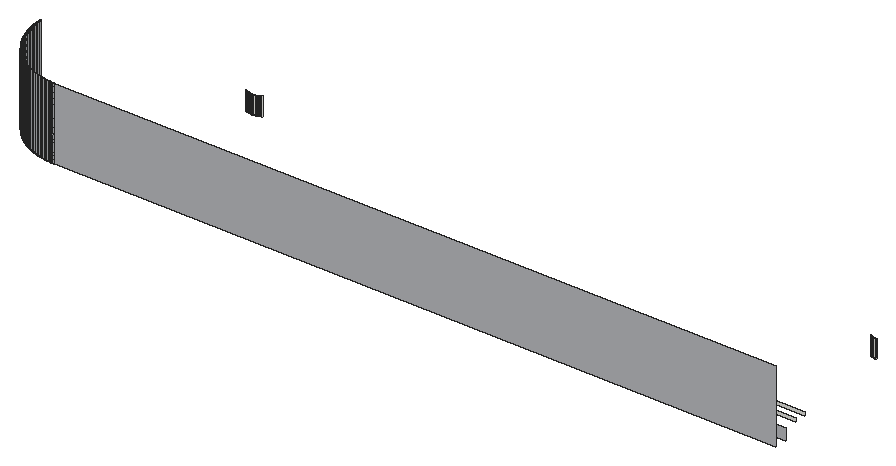
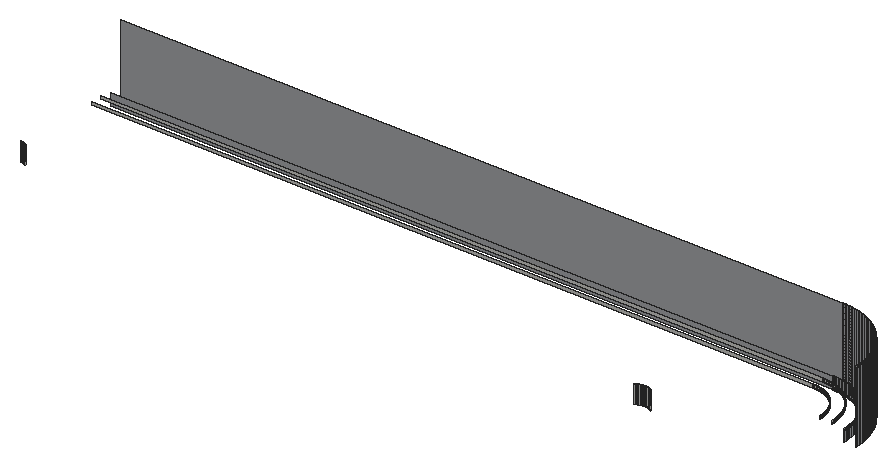
# SketchUp Ruby script. Lengths in inches.
U = 1.inch
M = Sketchup.active_model
def pt(a) = Geom::Point3d.new(a.map { |v| v * U })
def face(e, loops, mat)
  f = e.add_face(loops[0].map { |a| pt(a) })
  loops[1..].each { |l| e.add_face(l.map { |a| pt(a) }).erase! }
  f.material = f.back_material = mat if mat
  f
end
# faces: each face lists its corners as indices into pts; further lists are holes
def faces(e, pts, list, mat = nil) = list.each { |f| face(e, (f[0].is_a?(Array) ? f : [f]).map { |l| l.map { |i| pts[i] } }, mat) }
# xy, xz, yz: faces in a plane at the given z, y or x. An outline is a flat list of corners, or four numbers for a rectangle; further outlines are holes
def ring(l) = l.size == 4 ? [[l[0], l[1]], [l[2], l[1]], [l[2], l[3]], [l[0], l[3]]] : l.each_slice(2).to_a
def flat(e, list, mat, &to3) = list.each { |f| face(e, (f[0].is_a?(Array) ? f : [f]).map { |l| ring(l).map { |u, v| to3.(u, v) } }, mat) }
def xy(e, z, list, mat = nil) = flat(e, list, mat) { |x, y| [x, y, z] }
def xz(e, y, list, mat = nil) = flat(e, list, mat) { |x, z| [x, y, z] }
def yz(e, x, list, mat = nil) = flat(e, list, mat) { |y, z| [x, y, z] }
def lines(e, pts, list) = list.each { |a, b| e.add_line(pt(pts[a]), pt(pts[b])) }
# prism: a flat outline (further loops are holes) pulled along v
def prism(e, loops, v, mat = nil)
  f = face(e, loops, mat); d = Geom::Vector3d.new(v.map { |x| x * U })
  f.pushpull(f.normal.samedirection?(d) ? d.length : -d.length)
end
def box(e, o, s, mat = nil) = prism(e, [[o, [o[0] + s[0], o[1], o[2]], [o[0] + s[0], o[1] + s[1], o[2]], [o[0], o[1] + s[1], o[2]]]], [0, 0, s[2]], mat)
def at(x, y, z, deg = 0) = Geom::Transformation.translation(pt([x, y, z])) * Geom::Transformation.rotation(ORIGIN, Z_AXIS, deg.degrees)
def axes(o, x, y, z) = Geom::Transformation.new([*x, 0, *y, 0, *z, 0, *pt(o).to_a, 1])
def part(name) = M.definitions.add(name)
# library, detail: a bought-in or finely detailed component or shape, given as its bounding box
def library(name, o, s) = part(name).tap { |d| box(d.entities, o, s) }
def detail(e, o, s) = box(e.add_group.entities, o, s)
def put(e, d, t, mat = nil) = e.add_instance(d, t).tap { |i| i.material = mat if mat }
def group(e, t, mat = nil) = e.add_group.tap { |g| g.transformation = t; g.material = mat if mat }.entities
root = M.entities
M.materials.add("1427 AP 686 ARMOUR-N").color = [184, 186, 189]
xz(root,129.92,[[21,240,141,252]],"1427 AP 686 ARMOUR-N")
xz(root,129.93,[[20.53,240,20.6875,252],[20.6875,240,20.84,252]],"1427 AP 686 ARMOUR-N")
xz(root,131.92,[[21,240,21.01,242],[21.01,240,140.99,242]],"1427 AP 686 ARMOUR-N")
xz(root,131.93,[[20.61,240,20.74,242],[20.74,240,20.87,242]],"1427 AP 686 ARMOUR-N")
xz(root,133.92,[[21.01,242,140.99,242.5]])
xz(root,133.93,[[20.6875,242,20.79,242.5],[20.79,242,20.9,242.5]])
xz(root,133.94,[[20.48,242,20.58,242.5]])
xz(root,135.92,[[21.02,242,140.98,242.5]])
xz(root,135.93,[[20.6875,242,20.76,242.5],[20.76,242,20.84,242.5],[20.84,242,20.92,242.5]])
xz(root,153.43,[[34.84,242,34.92,245],[35.08,242,35.16,245]])
xz(root,153.44,[[34.6875,242,34.76,245],[35.24,242,35.3125,245],[138.6875,242,138.76,245]])
yz(root,9,[[141.61,240,141.77,252],[141.77,240,141.92,252]],"1427 AP 686 ARMOUR-N")
yz(root,11,[[141.66,240,141.79,242],[141.79,240,141.93,242]],"1427 AP 686 ARMOUR-N")
yz(root,11.01,[[141.4,240,141.53,242]],"1427 AP 686 ARMOUR-N")
yz(root,13,[[141.71,242,141.82,242.5],[141.82,242,141.9375,242.5]])
yz(root,13.01,[[141.51,242,141.61,242.5]])
yz(root,13.02,[[141.3,242,141.4,242.5]])
yz(root,15,[[141.6875,242,141.77,242.5],[141.77,242,141.85,242.5],[141.85,242,141.94,242.5]])
yz(root,15.01,[[141.53,242,141.61,242.5]])
yz(root,15.03,[[141.3,242,141.375,242.5]])
p = [[20.37,129.94,252],[20.22,129.95,252],[20.22,129.95,240],[20.37,129.94,240],[20.53,129.93,252],[20.53,129.93,240],
  [21,129.92,252],[20.84,129.93,252],[20.84,129.93,240],[20.99,129.92,240],[21,129.92,240],[19.28,130.05,252],
  [19.12,130.07,252],[19.12,130.07,240],[19.28,130.05,240],[19.43,130.03,252],[19.43,130.03,240],[19.59,130.01,252],
  [19.59,130.01,240],[19.75,129.99,252],[19.75,129.99,240],[19.9,129.97,252],[19.9,129.97,240],[20.06,129.96,252],
  [20.06,129.96,240],[18.8125,130.125,252],[18.66,130.15,252],[18.66,130.15,240],[18.8125,130.125,240],[18.97,130.1,252],
  [18.97,130.1,240],[18.35,130.22,252],[18.2,130.26,252],[18.2,130.26,240],[18.35,130.22,240],[18.51,130.1875,252],
  [18.51,130.1875,240],[17.89,130.33,252],[17.74,130.375,252],[17.74,130.375,240],[17.89,130.33,240],[18.05,130.29,252],
  [18.05,130.29,240],[17.59,130.42,252],[17.44,130.46,252],[17.44,130.46,240],[17.59,130.42,240],[17.29,130.51,252],
  [17.14,130.5625,252],[17.14,130.5625,240],[17.29,130.51,240],[16.99,130.61,252],[16.85,130.67,252],[16.85,130.67,240],
  [16.99,130.61,240],[16.7,130.72,252],[16.55,130.78,252],[16.55,130.78,240],[16.7,130.72,240],[16.41,130.84,252],
  [16.26,130.9,252],[16.26,130.9,240],[16.41,130.84,240],[16.12,130.96,252],[16.12,130.96,240],[15.98,131.03,252],
  [15.83,131.09,252],[15.83,131.09,240],[15.98,131.03,240],[15.69,131.16,252],[15.69,131.16,240],[15.55,131.23,252],
  [15.41,131.3,252],[15.41,131.3,240],[15.55,131.23,240],[15.27,131.38,252],[15.27,131.38,240],[15.14,131.45,252],
  [15.14,131.45,240],[15,131.53,252],[14.86,131.61,252],[14.86,131.61,240],[15,131.53,240],[14.73,131.69,252],
  [14.73,131.69,240],[14.6,131.78,252],[14.6,131.78,240],[14.46,131.86,252],[14.46,131.86,240],[14.33,131.95,252],
  [14.2,132.03,252],[14.2,132.03,240],[14.33,131.95,240],[20.35,131.95,240],[20.22,131.96,240],[20.22,131.96,242],
  [20.35,131.95,242],[20.48,131.9375,240],[20.48,131.9375,242],[20.61,131.93,240],[20.61,131.93,242],[21,131.92,240],
  [20.87,131.93,240],[20.87,131.93,242],[21,131.92,242],[14.07,132.125,252],[14.07,132.125,240],[19.4375,132.05,240],
  [19.31,132.07,240],[19.31,132.07,242],[19.4375,132.05,242],[19.57,132.03,240],[19.57,132.03,242],[19.69,132.01,240],
  [19.69,132.01,242],[19.82,131.99,240],[19.82,131.99,242],[19.95,131.98,240],[19.95,131.98,242],[20.09,131.97,240],
  [20.09,131.97,242],[13.95,132.22,252],[13.95,132.22,240],[18.92,132.14,240],[18.79,132.17,240],[18.79,132.17,242],
  [18.92,132.14,242],[19.05,132.12,240],[19.05,132.12,242],[19.18,132.09,240],[19.18,132.09,242],[13.82,132.31,252],
  [13.82,132.31,240],[18.54,132.23,240],[18.41,132.27,240],[18.41,132.27,242],[18.54,132.23,242],[18.67,132.2,240],
  [18.67,132.2,242],[13.69,132.4,252],[13.69,132.4,240],[18.16,132.34,240],[18.03,132.375,240],[18.03,132.375,242],
  [18.16,132.34,242],[18.29,132.3,240],[18.29,132.3,242],[13.57,132.5,252],[13.57,132.5,240],[17.91,132.41,240],
  [17.79,132.46,240],[17.79,132.46,242],[17.91,132.41,242],[13.45,132.6,252],[13.45,132.6,240],[17.54,132.54,240],
  [17.42,132.59,240],[17.42,132.59,242],[17.54,132.54,242],[17.66,132.5,240],[17.66,132.5,242],[13.33,132.7,252],
  [13.33,132.7,240],[17.29,132.64,240],[17.17,132.6875,240],[17.17,132.6875,242],[17.29,132.64,242],[13.21,132.8,252],
  [13.21,132.8,240],[17.05,132.74,240],[16.93,132.79,240],[16.93,132.79,242],[17.05,132.74,242],[13.09,132.9,252],
  [13.09,132.9,240],[16.8125,132.84,240],[16.7,132.9,240],[16.7,132.9,242],[16.8125,132.84,242],[12.97,133.01,252],
  [12.97,133.01,240],[16.58,132.96,240],[16.58,132.96,242],[12.85,133.11,252],[12.85,133.11,240],[16.46,133.01,240],
  [16.34,133.07,240],[16.34,133.07,242],[16.46,133.01,242],[12.74,133.22,252],[12.74,133.22,240],[16.23,133.14,240],
  [16.11,133.2,240],[16.11,133.2,242],[16.23,133.14,242],[12.625,133.33,252],[12.625,133.33,240],[16,133.26,240],
  [16,133.26,242],[12.51,133.4375,252],[12.51,133.4375,240],[15.89,133.33,240],[15.78,133.4,240],[15.78,133.4,242],
  [15.89,133.33,242],[12.4,133.55,252],[12.4,133.55,240],[15.66,133.47,240],[15.66,133.47,242],[15.55,133.54,240],
  [15.44,133.61,240],[15.44,133.61,242],[15.55,133.54,242],[12.3,133.66,252],[12.3,133.66,240],[15.34,133.68,240],
  [15.34,133.68,242],[12.1875,133.78,252],[12.1875,133.78,240],[15.23,133.76,240],[15.23,133.76,242],[12.08,133.89,252],
  [12.08,133.89,240],[15.12,133.83,240],[15.02,133.91,240],[15.02,133.91,242],[15.12,133.83,242],[11.98,134.01,252],
  [11.98,134.01,240],[14.91,133.99,240],[14.91,133.99,242],[11.875,134.13,252],[11.875,134.13,240],[14.81,134.07,240],
  [14.81,134.07,242],[11.77,134.25,252],[11.77,134.25,240],[14.71,134.15,240],[14.71,134.15,242],[14.61,134.24,240],
  [14.51,134.32,240],[14.51,134.32,242],[14.61,134.24,242],[11.67,134.37,252],[11.67,134.37,240],[14.41,134.41,240],
  [14.41,134.41,242],[11.58,134.5,252],[11.58,134.5,240],[14.31,134.49,240],[14.31,134.49,242],[11.48,134.62,252],
  [11.48,134.62,240],[14.21,134.58,240],[14.21,134.58,242],[11.39,134.74,252],[11.39,134.74,240],[14.12,134.67,240],
  [14.12,134.67,242],[11.29,134.87,252],[11.29,134.87,240],[14.02,134.76,240],[14.02,134.76,242],[13.93,134.85,240],
  [13.93,134.85,242],[11.2,135,252],[11.2,135,240],[13.84,134.95,240],[13.75,135.04,240],[13.75,135.04,242],
  [13.84,134.95,242],[11.11,135.13,252],[11.11,135.13,240],[13.66,135.14,240],[13.66,135.14,242],[11.02,135.26,252],
  [11.02,135.26,240],[13.57,135.23,240],[13.57,135.23,242],[13.48,135.33,240],[13.48,135.33,242],[10.9375,135.39,252],
  [10.9375,135.39,240],[13.4,135.43,240],[13.4,135.43,242],[10.85,135.52,252],[10.85,135.52,240],[13.3125,135.53,240],
  [13.3125,135.53,242],[10.77,135.65,252],[10.77,135.65,240],[13.23,135.63,240],[13.23,135.63,242],[13.15,135.73,240],
  [13.15,135.73,242],[10.6875,135.79,252],[10.6875,135.79,240],[13.07,135.84,240],[13.07,135.84,242],[10.61,135.92,252],
  [10.61,135.92,240],[12.99,135.94,240],[12.99,135.94,242],[10.53,136.0625,252],[10.53,136.0625,240],[12.91,136.05,240],
  [12.91,136.05,242],[12.83,136.15,240],[12.83,136.15,242],[10.45,136.2,252],[10.45,136.2,240],[10.38,136.34,252],
  [10.38,136.34,240],[12.76,136.26,240],[12.76,136.26,242],[10.31,136.48,252],[10.31,136.48,240],[12.69,136.37,240],
  [12.69,136.37,242],[12.61,136.48,240],[12.61,136.48,242],[10.24,136.62,252],[10.24,136.62,240],[12.54,136.59,240],
  [12.54,136.59,242],[10.17,136.76,252],[10.17,136.76,240],[12.47,136.7,240],[12.47,136.7,242],[12.41,136.8125,240],
  [12.41,136.8125,242],[10.1,136.9,252],[10.1,136.9,240],[12.34,136.92,240],[12.34,136.92,242],[10.04,137.04,252],
  [10.04,137.04,240],[12.28,137.04,240],[12.28,137.04,242],[9.97,137.1875,252],[9.97,137.1875,240],[12.21,137.15,240],
  [12.21,137.15,242],[9.91,137.33,252],[9.91,137.33,240],[12.15,137.27,240],[12.15,137.27,242],[9.85,137.48,252],
  [9.85,137.48,240],[12.09,137.38,240],[12.09,137.38,242],[12.03,137.5,240],[12.03,137.5,242],[9.8,137.625,252],
  [9.8,137.625,240],[11.97,137.62,240],[11.97,137.62,242],[9.74,137.77,252],[9.74,137.77,240],[11.92,137.74,240],
  [11.92,137.74,242],[11.86,137.86,240],[11.86,137.86,242],[9.6875,137.92,252],[9.6875,137.92,240],[9.64,138.07,252],
  [9.64,138.07,240],[11.8125,137.98,240],[11.8125,137.98,242],[11.76,138.1,240],[11.76,138.1,242],[9.59,138.22,252],
  [9.59,138.22,240],[11.71,138.22,240],[11.71,138.22,242],[9.54,138.37,252],[9.54,138.37,240],[11.66,138.34,240],
  [11.66,138.34,242],[11.62,138.46,240],[11.62,138.46,242],[9.49,138.52,252],[9.49,138.52,240],[9.45,138.67,252],
  [9.45,138.67,240],[11.57,138.59,240],[11.57,138.59,242],[11.53,138.71,240],[11.53,138.71,242],[9.41,138.82,252],
  [9.41,138.82,240],[11.49,138.83,240],[11.49,138.83,242],[9.37,138.97,252],[9.37,138.97,240],[11.45,138.96,240],
  [11.45,138.96,242],[9.33,139.125,252],[9.33,139.125,240],[11.41,139.08,240],[11.41,139.08,242],[9.3,139.28,252],
  [9.3,139.28,240],[11.375,139.21,240],[11.375,139.21,242],[11.34,139.34,240],[11.34,139.34,242],[9.26,139.43,252],
  [9.26,139.43,240],[11.31,139.46,240],[11.31,139.46,242],[9.23,139.58,252],[9.23,139.58,240],[11.28,139.59,240],
  [11.28,139.59,242],[9.2,139.74,252],[9.2,139.74,240],[11.25,139.72,240],[11.25,139.72,242],[9.17,139.89,252],
  [9.17,139.89,240],[11.22,139.85,240],[11.22,139.85,242],[11.19,139.97,240],[11.19,139.97,242],[9.15,140.05,252],
  [9.15,140.05,240],[9.125,140.2,252],[9.125,140.2,240],[11.17,140.1,240],[11.17,140.1,242],[11.14,140.23,240],
  [11.14,140.23,242],[9.1,140.36,252],[9.1,140.36,240],[11.125,140.36,240],[11.125,140.36,242],[9.08,140.51,252],
  [9.08,140.51,240],[11.1,140.49,240],[11.1,140.49,242],[9.07,140.67,252],[9.07,140.67,240],[11.09,140.62,240],
  [11.09,140.62,242],[11.07,140.75,240],[11.07,140.75,242],[9.05,140.83,252],[9.05,140.83,240],[11.05,140.88,240],
  [11.05,140.88,242],[9.04,140.98,252],[9.04,140.98,240],[11.04,141.01,240],[11.04,141.01,242],[9.03,141.14,252],
  [9.03,141.14,240],[11.03,141.14,240],[11.03,141.14,242],[9.02,141.3,252],[9.02,141.3,240],[11.02,141.27,240],
  [11.02,141.27,242],[9.01,141.45,252],[9.01,141.45,240],[11.01,141.4,240],[11.01,141.4,242],[9,141.61,252],
  [9,141.61,240],[11.01,141.53,240],[11,141.66,240],[11,141.66,242],[11.01,141.53,242],[20.37,133.95,242],
  [20.27,133.96,242],[20.27,133.96,242.5],[20.37,133.95,242.5],[20.48,133.94,242],[20.48,133.94,242.5],[20.6875,133.93,242],
  [20.58,133.94,242],[20.58,133.94,242.5],[20.6875,133.93,242.5],[21.01,133.92,242],[20.9,133.93,242],[20.9,133.93,242.5],
  [21.01,133.92,242.5],[19.65,134.04,242],[19.54,134.06,242],[19.54,134.06,242.5],[19.65,134.04,242.5],[19.75,134.02,242],
  [19.75,134.02,242.5],[19.85,134.01,242],[19.85,134.01,242.5],[19.96,133.99,242],[19.96,133.99,242.5],[20.06,133.98,242],
  [20.06,133.98,242.5],[20.16,133.97,242],[20.16,133.97,242.5],[19.13,134.15,242],[19.03,134.17,242],[19.03,134.17,242.5],
  [19.13,134.15,242.5],[19.23,134.12,242],[19.23,134.12,242.5],[19.34,134.1,242],[19.34,134.1,242.5],[19.4375,134.08,242],
  [19.4375,134.08,242.5],[18.83,134.22,242],[18.73,134.25,242],[18.73,134.25,242.5],[18.83,134.22,242.5],[18.93,134.2,242],
  [18.93,134.2,242.5],[18.43,134.35,242],[18.33,134.38,242],[18.33,134.38,242.5],[18.43,134.35,242.5],[18.53,134.32,242],
  [18.53,134.32,242.5],[18.63,134.28,242],[18.63,134.28,242.5],[18.23,134.42,242],[18.13,134.46,242],[18.13,134.46,242.5],
  [18.23,134.42,242.5],[17.9375,134.53,242],[17.84,134.57,242],[17.84,134.57,242.5],[17.9375,134.53,242.5],[18.04,134.49,242],
  [18.04,134.49,242.5],[17.75,134.62,242],[17.65,134.66,242],[17.65,134.66,242.5],[17.75,134.62,242.5],[17.46,134.75,242],
  [17.37,134.8,242],[17.37,134.8,242.5],[17.46,134.75,242.5],[17.56,134.7,242],[17.56,134.7,242.5],[17.28,134.84,242],
  [17.18,134.89,242],[17.18,134.89,242.5],[17.28,134.84,242.5],[17.09,134.94,242],[17,135,242],[17,135,242.5],
  [17.09,134.94,242.5],[16.91,135.05,242],[16.82,135.1,242],[16.82,135.1,242.5],[16.91,135.05,242.5],[16.73,135.16,242],
  [16.73,135.16,242.5],[16.64,135.22,242],[16.56,135.27,242],[16.56,135.27,242.5],[16.64,135.22,242.5],[16.47,135.33,242],
  [16.38,135.39,242],[16.38,135.39,242.5],[16.47,135.33,242.5],[16.3,135.45,242],[16.3,135.45,242.5],[16.21,135.51,242],
  [16.13,135.58,242],[16.13,135.58,242.5],[16.21,135.51,242.5],[16.05,135.64,242],[15.97,135.71,242],[15.97,135.71,242.5],
  [16.05,135.64,242.5],[15.88,135.77,242],[15.88,135.77,242.5],[15.8,135.84,242],[15.73,135.91,242],[15.73,135.91,242.5],
  [15.8,135.84,242.5],[15.65,135.98,242],[15.65,135.98,242.5],[20.37,135.96,242],[20.45,135.95,242],[20.45,135.95,242.5],
  [20.37,135.96,242.5],[20.53,135.94,242],[20.53,135.94,242.5],[20.61,135.9375,242],[20.61,135.9375,242.5],[20.6875,135.93,242],
  [20.6875,135.93,242.5],[20.92,135.93,242],[21.02,135.92,242],[21.02,135.92,242.5],[20.92,135.93,242.5],[15.57,136.05,242],
  [15.49,136.12,242],[15.49,136.12,242.5],[15.57,136.05,242.5],[19.75,136.06,242],[19.83,136.04,242],[19.83,136.04,242.5],
  [19.75,136.06,242.5],[19.91,136.02,242],[19.91,136.02,242.5],[19.98,136.01,242],[19.98,136.01,242.5],[20.0625,136,242],
  [20.0625,136,242.5],[20.14,135.99,242],[20.14,135.99,242.5],[20.22,135.98,242],[20.22,135.98,242.5],[20.29,135.97,242],
  [20.29,135.97,242.5],[15.42,136.19,242],[15.42,136.19,242.5],[19.3,136.17,242],[19.37,136.15,242],[19.37,136.15,242.5],
  [19.3,136.17,242.5],[19.45,136.13,242],[19.45,136.13,242.5],[19.52,136.11,242],[19.52,136.11,242.5],[19.6,136.09,242],
  [19.6,136.09,242.5],[19.68,136.07,242],[19.68,136.07,242.5],[15.34,136.27,242],[15.34,136.27,242.5],[19,136.27,242],
  [19.07,136.24,242],[19.07,136.24,242.5],[19,136.27,242.5],[19.15,136.22,242],[19.15,136.22,242.5],[19.22,136.19,242],
  [19.22,136.19,242.5],[15.27,136.34,242],[15.2,136.42,242],[15.2,136.42,242.5],[15.27,136.34,242.5],[18.78,136.35,242],
  [18.85,136.32,242],[18.85,136.32,242.5],[18.78,136.35,242.5],[18.92,136.3,242],[18.92,136.3,242.5],[15.125,136.49,242],
  [15.125,136.49,242.5],[18.49,136.48,242],[18.56,136.44,242],[18.56,136.44,242.5],[18.49,136.48,242.5],[18.63,136.41,242],
  [18.63,136.41,242.5],[18.7,136.38,242],[18.7,136.38,242.5],[15.05,136.57,242],[15.05,136.57,242.5],[18.28,136.58,242],
  [18.35,136.54,242],[18.35,136.54,242.5],[18.28,136.58,242.5],[18.42,136.51,242],[18.42,136.51,242.5],[14.99,136.65,242],
  [14.92,136.73,242],[14.92,136.73,242.5],[14.99,136.65,242.5],[18.14,136.65,242],[18.21,136.61,242],[18.21,136.61,242.5],
  [18.14,136.65,242.5],[14.85,136.81,242],[14.85,136.81,242.5],[17.93,136.77,242],[18,136.73,242],[18,136.73,242.5],
  [17.93,136.77,242.5],[18.07,136.69,242],[18.07,136.69,242.5],[14.78,136.89,242],[14.78,136.89,242.5],[17.8,136.85,242],
  [17.87,136.81,242],[17.87,136.81,242.5],[17.8,136.85,242.5],[14.72,136.97,242],[14.72,136.97,242.5],[17.6,136.98,242],
  [17.67,136.9375,242],[17.67,136.9375,242.5],[17.6,136.98,242.5],[17.73,136.89,242],[17.73,136.89,242.5],[14.65,137.05,242],
  [14.65,137.05,242.5],[17.47,137.07,242],[17.54,137.02,242],[17.54,137.02,242.5],[17.47,137.07,242.5],[14.59,137.14,242],
  [14.53,137.22,242],[14.53,137.22,242.5],[14.59,137.14,242.5],[17.35,137.16,242],[17.41,137.12,242],[17.41,137.12,242.5],
  [17.35,137.16,242.5],[14.47,137.31,242],[14.47,137.31,242.5],[17.22,137.26,242],[17.29,137.21,242],[17.29,137.21,242.5],
  [17.22,137.26,242.5],[14.41,137.39,242],[14.41,137.39,242.5],[17.1,137.36,242],[17.16,137.3125,242],[17.16,137.3125,242.5],
  [17.1,137.36,242.5],[14.35,137.48,242],[14.35,137.48,242.5],[16.99,137.47,242],[17.04,137.41,242],[17.04,137.41,242.5],
  [16.99,137.47,242.5],[14.29,137.57,242],[14.29,137.57,242.5],[16.87,137.57,242],[16.93,137.52,242],[16.93,137.52,242.5],
  [16.87,137.57,242.5],[14.23,137.66,242],[14.23,137.66,242.5],[16.76,137.68,242],[16.8125,137.625,242],[16.8125,137.625,242.5],
  [16.76,137.68,242.5],[14.18,137.74,242],[14.125,137.83,242],[14.125,137.83,242.5],[14.18,137.74,242.5],[16.65,137.79,242],
  [16.7,137.74,242],[16.7,137.74,242.5],[16.65,137.79,242.5],[14.07,137.92,242],[14.07,137.92,242.5],[16.59,137.85,242],
  [16.59,137.85,242.5],[14.02,138.02,242],[14.02,138.02,242.5],[16.49,137.97,242],[16.54,137.91,242],[16.54,137.91,242.5],
  [16.49,137.97,242.5],[13.97,138.11,242],[13.97,138.11,242.5],[16.39,138.09,242],[16.4375,138.03,242],[16.4375,138.03,242.5],
  [16.39,138.09,242.5],[13.92,138.2,242],[13.92,138.2,242.5],[16.29,138.21,242],[16.34,138.15,242],[16.34,138.15,242.5],
  [16.29,138.21,242.5],[13.87,138.29,242],[13.87,138.29,242.5],[16.24,138.27,242],[16.24,138.27,242.5],[13.83,138.39,242],
  [13.83,138.39,242.5],[16.15,138.4,242],[16.19,138.33,242],[16.19,138.33,242.5],[16.15,138.4,242.5],[13.78,138.48,242],
  [13.78,138.48,242.5],[16.1,138.46,242],[16.1,138.46,242.5],[13.74,138.58,242],[13.74,138.58,242.5],[16.01,138.59,242],
  [16.06,138.53,242],[16.06,138.53,242.5],[16.01,138.59,242.5],[13.69,138.67,242],[13.69,138.67,242.5],[15.97,138.66,242],
  [15.97,138.66,242.5],[13.65,138.77,242],[13.65,138.77,242.5],[15.88,138.79,242],[15.93,138.72,242],[15.93,138.72,242.5],
  [15.88,138.79,242.5],[13.61,138.86,242],[13.61,138.86,242.5],[15.84,138.86,242],[15.84,138.86,242.5],[13.57,138.96,242],
  [13.57,138.96,242.5],[15.77,138.99,242],[15.8,138.92,242],[15.8,138.92,242.5],[15.77,138.99,242.5],[13.53,139.06,242],
  [13.53,139.06,242.5],[15.73,139.0625,242],[15.73,139.0625,242.5],[13.49,139.16,242],[13.49,139.16,242.5],[15.65,139.2,242],
  [15.69,139.13,242],[15.69,139.13,242.5],[15.65,139.2,242.5],[13.46,139.25,242],[13.46,139.25,242.5],[15.62,139.27,242],
  [15.62,139.27,242.5],[13.42,139.35,242],[13.42,139.35,242.5],[15.55,139.41,242],[15.58,139.34,242],[15.58,139.34,242.5],
  [15.55,139.41,242.5],[13.39,139.45,242],[13.39,139.45,242.5],[15.52,139.48,242],[15.52,139.48,242.5],[13.36,139.55,242],
  [13.36,139.55,242.5],[15.49,139.56,242],[15.49,139.56,242.5],[13.33,139.65,242],[13.33,139.65,242.5],[15.43,139.7,242],
  [15.46,139.63,242],[15.46,139.63,242.5],[15.43,139.7,242.5],[13.3,139.75,242],[13.3,139.75,242.5],[15.4,139.77,242],
  [15.4,139.77,242.5],[13.27,139.85,242],[13.27,139.85,242.5],[15.34,139.92,242],[15.37,139.85,242],[15.37,139.85,242.5],
  [15.34,139.92,242.5],[13.25,139.96,242],[13.25,139.96,242.5],[15.32,140,242],[15.32,140,242.5],[13.22,140.06,242],
  [13.22,140.06,242.5],[15.29,140.07,242],[15.29,140.07,242.5],[13.2,140.16,242],[13.2,140.16,242.5],[15.25,140.22,242],
  [15.27,140.15,242],[15.27,140.15,242.5],[15.25,140.22,242.5],[13.17,140.26,242],[13.17,140.26,242.5],[15.23,140.3,242],
  [15.23,140.3,242.5],[13.15,140.36,242],[13.15,140.36,242.5],[15.2,140.37,242],[15.2,140.37,242.5],[13.13,140.47,242],
  [13.13,140.47,242.5],[15.17,140.52,242],[15.18,140.45,242],[15.18,140.45,242.5],[15.17,140.52,242.5],[13.12,140.57,242],
  [13.12,140.57,242.5],[15.15,140.6,242],[15.15,140.6,242.5],[13.1,140.67,242],[13.1,140.67,242.5],[15.13,140.68,242],
  [15.13,140.68,242.5],[13.08,140.78,242],[13.08,140.78,242.5],[15.12,140.75,242],[15.12,140.75,242.5],[13.07,140.88,242],
  [13.07,140.88,242.5],[15.09,140.91,242],[15.1,140.83,242],[15.1,140.83,242.5],[15.09,140.91,242.5],[13.06,140.98,242],
  [13.06,140.98,242.5],[15.07,140.99,242],[15.07,140.99,242.5],[13.04,141.09,242],[13.04,141.09,242.5],[15.0625,141.0625,242],
  [15.0625,141.0625,242.5],[13.03,141.19,242],[13.03,141.19,242.5],[15.04,141.22,242],[15.05,141.14,242],[15.05,141.14,242.5],
  [15.04,141.22,242.5],[13.02,141.3,242],[13.02,141.3,242.5],[15.03,141.3,242],[15.03,141.3,242.5],[13.02,141.4,242],
  [13.01,141.51,242],[13.01,141.51,242.5],[13.02,141.4,242.5],[15.02,141.45,242],[15.03,141.375,242],[15.03,141.375,242.5],
  [15.02,141.45,242.5],[15.01,141.53,242],[15.01,141.53,242.5],[13.01,141.61,242],[13,141.71,242],[13,141.71,242.5],
  [13.01,141.61,242.5],[15,141.6875,242],[15.01,141.61,242],[15.01,141.61,242.5],[15,141.6875,242.5],[34.6875,153.44,242],
  [34.61,153.46,242],[34.61,153.46,245],[34.6875,153.44,245],[34.84,153.43,242],[34.76,153.44,242],[34.76,153.44,245],
  [34.84,153.43,245],[35,153.42,242],[34.92,153.43,242],[34.92,153.43,245],[35,153.42,245],[35.08,153.43,242],
  [35.08,153.43,245],[35.24,153.44,242],[35.16,153.43,242],[35.16,153.43,245],[35.24,153.44,245],[35.39,153.46,242],
  [35.3125,153.44,242],[35.3125,153.44,245],[35.39,153.46,245],[138.6875,153.44,242],[138.61,153.46,242],[138.61,153.46,245],
  [138.6875,153.44,245],[138.84,153.43,242],[138.76,153.44,242],[138.76,153.44,245],[138.84,153.43,245],[34.23,153.55,242],
  [34.15,153.57,242],[34.15,153.57,245],[34.23,153.55,245],[34.3,153.52,242],[34.3,153.52,245],[34.38,153.5,242],
  [34.38,153.5,245],[34.45,153.48,242],[34.45,153.48,245],[34.53,153.47,242],[34.53,153.47,245],[35.47,153.47,242],
  [35.47,153.47,245],[35.55,153.48,242],[35.55,153.48,245],[35.62,153.5,242],[35.62,153.5,245],[35.7,153.52,242],
  [35.7,153.52,245],[35.77,153.55,242],[35.77,153.55,245],[35.85,153.57,242],[35.85,153.57,245],[138.23,153.55,242],
  [138.15,153.57,242],[138.15,153.57,245],[138.23,153.55,245],[138.3,153.52,242],[138.3,153.52,245],[138.38,153.5,242],
  [138.38,153.5,245],[138.45,153.48,242],[138.45,153.48,245],[138.53,153.47,242],[138.53,153.47,245],[34.01,153.63,242],
  [33.9375,153.66,242],[33.9375,153.66,245],[34.01,153.63,245],[34.08,153.6,242],[34.08,153.6,245],[35.92,153.6,242],
  [35.92,153.6,245],[35.99,153.63,242],[35.99,153.63,245],[36.06,153.66,242],[36.06,153.66,245],[138.01,153.63,242],
  [137.9375,153.66,242],[137.9375,153.66,245],[138.01,153.63,245],[138.08,153.6,242],[138.08,153.6,245],[33.8,153.73,242],
  [33.73,153.77,242],[33.73,153.77,245],[33.8,153.73,245],[33.87,153.7,242],[33.87,153.7,245],[36.14,153.7,242],
  [36.14,153.7,245],[36.2,153.73,242],[36.2,153.73,245],[36.27,153.77,242],[36.27,153.77,245],[137.8,153.73,242],
  [137.73,153.77,242],[137.73,153.77,245],[137.8,153.73,245],[137.87,153.7,242],[137.87,153.7,245],[33.66,153.8125,242],
  [33.59,153.86,242],[33.59,153.86,245],[33.66,153.8125,245],[36.34,153.8125,242],[36.34,153.8125,245],[36.41,153.86,242],
  [36.41,153.86,245],[137.66,153.8125,242],[137.66,153.8125,245]]
faces(root,p,[[0,1,2,3],[4,0,3,5],[6,7,8,9,10],[11,12,13,14],[15,11,14,16],[17,15,16,18],[19,17,18,20],[21,19,20,22],
  [23,21,22,24],[1,23,24,2],[25,26,27,28],[29,25,28,30],[12,29,30,13],[31,32,33,34],[35,31,34,36],[26,35,36,27],
  [37,38,39,40],[41,37,40,42],[32,41,42,33],[43,44,45,46],[38,43,46,39],[47,48,49,50],[44,47,50,45],[51,52,53,54],
  [48,51,54,49],[55,56,57,58],[52,55,58,53],[59,60,61,62],[56,59,62,57],[60,63,64,61],[65,66,67,68],[63,65,68,64],
  [66,69,70,67],[71,72,73,74],[69,71,74,70],[72,75,76,73],[75,77,78,76],[79,80,81,82],[77,79,82,78],[80,83,84,81],
  [83,85,86,84],[85,87,88,86],[89,90,91,92],[87,89,92,88],[93,94,95,96],[97,93,96,98],[99,97,98,100],[101,102,103,104],
  [90,105,106,91],[107,108,109,110],[111,107,110,112],[113,111,112,114],[115,113,114,116],[117,115,116,118],[119,117,118,120],[94,119,120,95],
  [105,121,122,106],[123,124,125,126],[127,123,126,128],[129,127,128,130],[108,129,130,109],[121,131,132,122],[133,134,135,136],[137,133,136,138],
  [124,137,138,125],[131,139,140,132],[141,142,143,144],[145,141,144,146],[134,145,146,135],[139,147,148,140],[149,150,151,152],[142,149,152,143],
  [147,153,154,148],[155,156,157,158],[159,155,158,160],[150,159,160,151],[153,161,162,154],[163,164,165,166],[156,163,166,157],[161,167,168,162],
  [169,170,171,172],[164,169,172,165],[167,173,174,168],[175,176,177,178],[170,175,178,171],[173,179,180,174],[176,181,182,177],[179,183,184,180],
  [185,186,187,188],[181,185,188,182],[183,189,190,184],[191,192,193,194],[186,191,194,187],[189,195,196,190],[192,197,198,193],[195,199,200,196],
  [201,202,203,204],[197,201,204,198],[199,205,206,200],[202,207,208,203],[209,210,211,212],[207,209,212,208],[205,213,214,206],[210,215,216,211],
  [213,217,218,214],[215,219,220,216],[217,221,222,218],[223,224,225,226],[219,223,226,220],[221,227,228,222],[224,229,230,225],[227,231,232,228],
  [229,233,234,230],[231,235,236,232],[233,237,238,234],[239,240,241,242],[237,239,242,238],[235,243,244,236],[240,245,246,241],[243,247,248,244],
  [245,249,250,246],[247,251,252,248],[249,253,254,250],[251,255,256,252],[253,257,258,254],[255,259,260,256],[257,261,262,258],[261,263,264,262],
  [259,265,266,260],[267,268,269,270],[263,267,270,264],[265,271,272,266],[268,273,274,269],[271,275,276,272],[273,277,278,274],[277,279,280,278],
  [275,281,282,276],[279,283,284,280],[281,285,286,282],[283,287,288,284],[285,289,290,286],[287,291,292,288],[291,293,294,292],[289,295,296,290],
  [293,297,298,294],[295,299,300,296],[297,301,302,298],[299,303,304,300],[301,305,306,302],[305,307,308,306],[303,309,310,304],[309,311,312,310],
  [307,313,314,308],[311,315,316,312],[313,317,318,314],[317,319,320,318],[315,321,322,316],[319,323,324,320],[321,325,326,322],[323,327,328,324],
  [327,329,330,328],[325,331,332,326],[329,333,334,330],[331,335,336,332],[333,337,338,334],[335,339,340,336],[337,341,342,338],[339,343,344,340],
  [341,345,346,342],[343,347,348,344],[345,349,350,346],[349,351,352,350],[347,353,354,348],[351,355,356,352],[353,357,358,354],[355,359,360,356],
  [359,361,362,360],[357,363,364,358],[363,365,366,364],[361,367,368,362],[367,369,370,368],[365,371,372,366],[369,373,374,370],[371,375,376,372],
  [373,377,378,374],[377,379,380,378],[375,381,382,376],[381,383,384,382],[379,385,386,380],[385,387,388,386],[383,389,390,384],[387,391,392,388],
  [389,393,394,390],[391,395,396,392],[393,397,398,394],[395,399,400,396],[397,401,402,398],[399,403,404,400],[403,405,406,404],[401,407,408,402],
  [405,409,410,406],[407,411,412,408],[409,413,414,410],[411,415,416,412],[413,417,418,414],[415,419,420,416],[417,421,422,418],[421,423,424,422],
  [419,425,426,420],[425,427,428,426],[423,429,430,424],[429,431,432,430],[427,433,434,428],[431,435,436,432],[433,437,438,434],[435,439,440,436],
  [437,441,442,438],[439,443,444,440],[443,445,446,444],[441,447,448,442],[445,449,450,446],[447,451,452,448],[449,453,454,450],[451,455,456,452],
  [453,457,458,454],[455,459,460,456],[457,461,462,458],[459,463,464,460],[461,465,466,462],[463,467,468,464],[469,470,471,472]],"1427 AP 686 ARMOUR-N")
faces(root,p,[[473,474,475,476],[477,473,476,478],[479,480,481,482],[483,484,485,486],[487,488,489,490],[491,487,490,492],[493,491,492,494],[495,493,494,496],
  [497,495,496,498],[499,497,498,500],[474,499,500,475],[501,502,503,504],[505,501,504,506],[507,505,506,508],[509,507,508,510],[488,509,510,489],
  [511,512,513,514],[515,511,514,516],[502,515,516,503],[517,518,519,520],[521,517,520,522],[523,521,522,524],[512,523,524,513],[525,526,527,528],
  [518,525,528,519],[529,530,531,532],[533,529,532,534],[526,533,534,527],[535,536,537,538],[530,535,538,531],[539,540,541,542],[543,539,542,544],
  [536,543,544,537],[545,546,547,548],[540,545,548,541],[549,550,551,552],[546,549,552,547],[553,554,555,556],[550,553,556,551],[554,557,558,555],
  [559,560,561,562],[557,559,562,558],[563,564,565,566],[560,563,566,561],[564,567,568,565],[569,570,571,572],[567,569,572,568],[573,574,575,576],
  [570,573,576,571],[574,577,578,575],[579,580,581,582],[577,579,582,578],[580,583,584,581],[585,586,587,588],[586,589,590,587],[589,591,592,590],
  [591,593,594,592],[595,596,597,598],[599,600,601,602],[583,599,602,584],[603,604,605,606],[604,607,608,605],[607,609,610,608],[609,611,612,610],
  [611,613,614,612],[613,615,616,614],[615,617,618,616],[617,585,588,618],[600,619,620,601],[621,622,623,624],[622,625,626,623],[625,627,628,626],
  [627,629,630,628],[629,631,632,630],[631,603,606,632],[619,633,634,620],[635,636,637,638],[636,639,640,637],[639,641,642,640],[641,621,624,642],
  [643,644,645,646],[633,643,646,634],[647,648,649,650],[648,651,652,649],[651,635,638,652],[644,653,654,645],[655,656,657,658],[656,659,660,657],
  [659,661,662,660],[661,647,650,662],[653,663,664,654],[665,666,667,668],[666,669,670,667],[669,655,658,670],[671,672,673,674],[663,671,674,664],
  [675,676,677,678],[676,665,668,677],[672,679,680,673],[681,682,683,684],[682,685,686,683],[685,675,678,686],[679,687,688,680],[689,690,691,692],
  [690,681,684,691],[687,693,694,688],[695,696,697,698],[696,699,700,697],[699,689,692,700],[693,701,702,694],[703,704,705,706],[704,695,698,705],
  [707,708,709,710],[701,707,710,702],[711,712,713,714],[712,703,706,713],[708,715,716,709],[717,718,719,720],[718,711,714,719],[715,721,722,716],
  [723,724,725,726],[724,717,720,725],[721,727,728,722],[729,730,731,732],[730,723,726,731],[727,733,734,728],[735,736,737,738],[736,729,732,737],
  [733,739,740,734],[741,742,743,744],[742,735,738,743],[745,746,747,748],[739,745,748,740],[749,750,751,752],[750,741,744,751],[746,753,754,747],
  [755,749,752,756],[753,757,758,754],[759,760,761,762],[760,755,756,761],[757,763,764,758],[765,766,767,768],[766,759,762,767],[763,769,770,764],
  [771,772,773,774],[772,765,768,773],[769,775,776,770],[777,771,774,778],[775,779,780,776],[781,782,783,784],[782,777,778,783],[779,785,786,780],
  [787,781,784,788],[785,789,790,786],[791,792,793,794],[792,787,788,793],[789,795,796,790],[797,791,794,798],[795,799,800,796],[801,802,803,804],
  [802,797,798,803],[799,805,806,800],[807,801,804,808],[805,809,810,806],[811,812,813,814],[812,807,808,813],[809,815,816,810],[817,811,814,818],
  [815,819,820,816],[821,822,823,824],[822,817,818,823],[819,825,826,820],[827,821,824,828],[825,829,830,826],[831,832,833,834],[832,827,828,833],
  [829,835,836,830],[837,831,834,838],[835,839,840,836],[841,837,838,842],[839,843,844,840],[845,846,847,848],[846,841,842,847],[843,849,850,844],
  [851,845,848,852],[849,853,854,850],[855,856,857,858],[856,851,852,857],[853,859,860,854],[861,855,858,862],[859,863,864,860],[865,861,862,866],
  [863,867,868,864],[869,870,871,872],[870,865,866,871],[867,873,874,868],[875,869,872,876],[873,877,878,874],[879,875,876,880],[877,881,882,878],
  [883,884,885,886],[884,879,880,885],[881,887,888,882],[889,883,886,890],[887,891,892,888],[893,889,890,894],[891,895,896,892],[897,893,894,898],
  [895,899,900,896],[901,902,903,904],[902,897,898,903],[899,905,906,900],[907,901,904,908],[905,909,910,906],[911,907,908,912],[909,913,914,910],
  [915,916,917,918],[916,911,912,917],[913,919,920,914],[921,915,918,922],[923,924,925,926],[927,928,929,930],[931,927,930,932],[933,934,935,936],
  [937,938,939,940],[941,942,943,944],[945,946,947,948],[949,950,951,952],[953,949,952,954],[955,956,957,958],[959,960,961,962],[963,964,965,966],
  [967,968,969,970],[971,972,973,974],[975,971,974,976],[977,975,976,978],[979,977,978,980],[981,979,980,982],[942,981,982,943],[983,959,962,984],
  [985,983,984,986],[987,985,986,988],[989,987,988,990],[991,989,990,992],[993,991,992,994],[995,996,997,998],[999,995,998,1000],[1001,999,1000,1002],
  [1003,1001,1002,1004],[1005,1003,1004,1006],[964,1005,1006,965],[1007,1008,1009,1010],[1011,1007,1010,1012],[972,1011,1012,973],[1013,993,994,1014],[1015,1013,1014,1016],
  [1017,1015,1016,1018],[1019,1020,1021,1022],[1023,1019,1022,1024],[996,1023,1024,997],[1025,1026,1027,1028],[1029,1025,1028,1030],[1008,1029,1030,1009],[1031,1017,1018,1032],
  [1033,1031,1032,1034],[1035,1033,1034,1036],[1037,1038,1039,1040],[1041,1037,1040,1042],[1020,1041,1042,1021],[1043,1044,1045,1046],[1026,1043,1046,1027],[1047,1035,1036,1048],
  [1049,1047,1048,1050],[1038,1051,1052,1039]])
